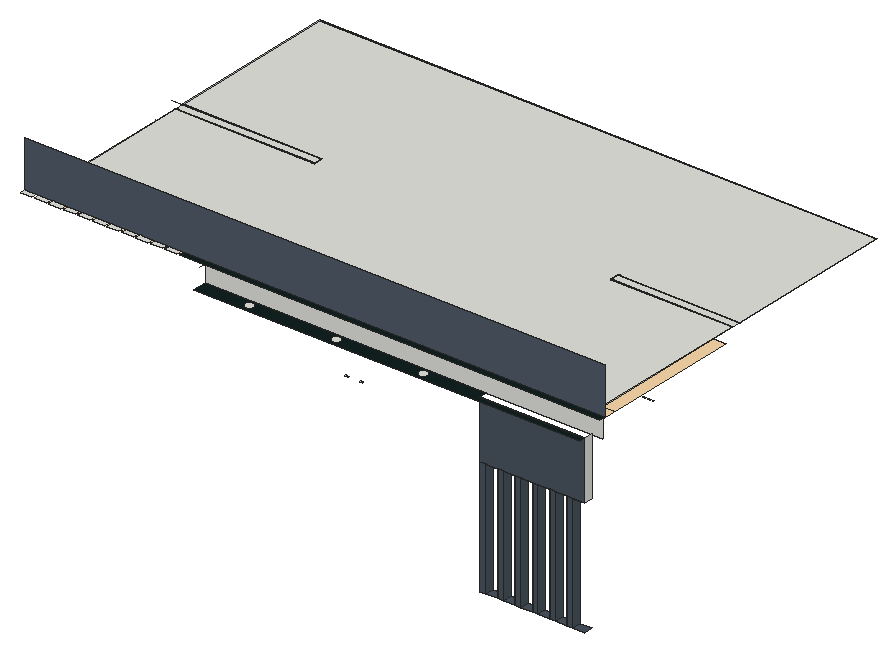
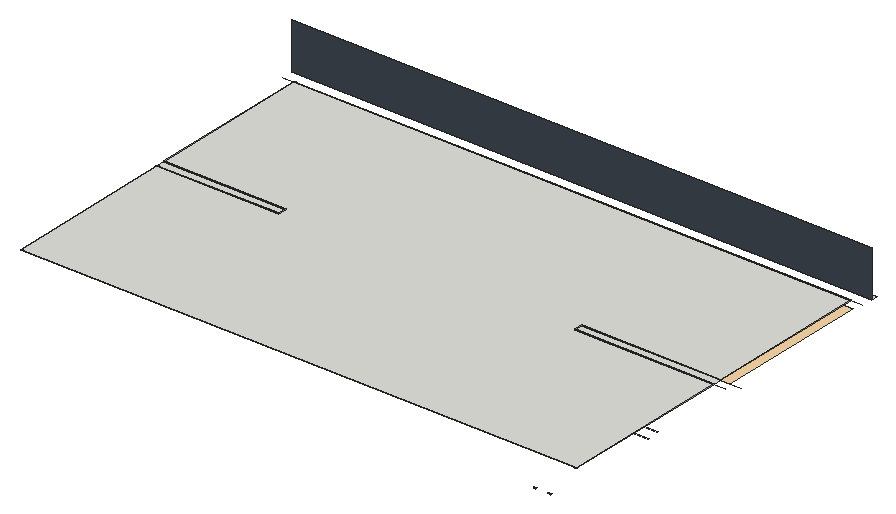
# SketchUp Ruby script. Lengths in millimetres.
U = 1.mm
M = Sketchup.active_model
def pt(a) = Geom::Point3d.new(a.map { |v| v * U })
def face(e, loops, mat)
  f = e.add_face(loops[0].map { |a| pt(a) })
  loops[1..].each { |l| e.add_face(l.map { |a| pt(a) }).erase! }
  f.material = f.back_material = mat if mat
  f
end
# faces: each face lists its corners as indices into pts; further lists are holes
def faces(e, pts, list, mat = nil) = list.each { |f| face(e, (f[0].is_a?(Array) ? f : [f]).map { |l| l.map { |i| pts[i] } }, mat) }
# xy, xz, yz: faces in a plane at the given z, y or x. An outline is a flat list of corners, or four numbers for a rectangle; further outlines are holes
def ring(l) = l.size == 4 ? [[l[0], l[1]], [l[2], l[1]], [l[2], l[3]], [l[0], l[3]]] : l.each_slice(2).to_a
def flat(e, list, mat, &to3) = list.each { |f| face(e, (f[0].is_a?(Array) ? f : [f]).map { |l| ring(l).map { |u, v| to3.(u, v) } }, mat) }
def xy(e, z, list, mat = nil) = flat(e, list, mat) { |x, y| [x, y, z] }
def xz(e, y, list, mat = nil) = flat(e, list, mat) { |x, z| [x, y, z] }
def yz(e, x, list, mat = nil) = flat(e, list, mat) { |y, z| [x, y, z] }
def lines(e, pts, list) = list.each { |a, b| e.add_line(pt(pts[a]), pt(pts[b])) }
# prism: a flat outline (further loops are holes) pulled along v
def prism(e, loops, v, mat = nil)
  f = face(e, loops, mat); d = Geom::Vector3d.new(v.map { |x| x * U })
  f.pushpull(f.normal.samedirection?(d) ? d.length : -d.length)
end
def box(e, o, s, mat = nil) = prism(e, [[o, [o[0] + s[0], o[1], o[2]], [o[0] + s[0], o[1] + s[1], o[2]], [o[0], o[1] + s[1], o[2]]]], [0, 0, s[2]], mat)
def at(x, y, z, deg = 0) = Geom::Transformation.translation(pt([x, y, z])) * Geom::Transformation.rotation(ORIGIN, Z_AXIS, deg.degrees)
def axes(o, x, y, z) = Geom::Transformation.new([*x, 0, *y, 0, *z, 0, *pt(o).to_a, 1])
def part(name) = M.definitions.add(name)
# library, detail: a bought-in or finely detailed component or shape, given as its bounding box
def library(name, o, s) = part(name).tap { |d| box(d.entities, o, s) }
def detail(e, o, s) = box(e.add_group.entities, o, s)
def put(e, d, t, mat = nil) = e.add_instance(d, t).tap { |i| i.material = mat if mat }
def group(e, t, mat = nil) = e.add_group.tap { |g| g.transformation = t; g.material = mat if mat }.entities
root = M.entities
M.materials.add("[0033_NavajoWhite]").color = [249, 217, 169]
M.materials.add("[0078_DarkSlateGray]").color = [19, 33, 33]
M.materials.add("[0110_LightSlateGray]").color = [73, 83, 94]
M.materials.add("[0111_SlateGray]").color = [81, 92, 104]
xy(root,54270.3,[[31307.7,14109.7,31917.3,14566.9],[32222.1,14109.7,32831.7,14566.9],[33136.5,14109.7,33746.1,14566.9],[34050.9,14109.7,34660.5,14566.9],[34965.3,14109.7,35574.9,14566.9],
  [35879.7,14109.7,36489.3,14566.9]],"[0110_LightSlateGray]")
xy(root,55822.5,[[17116.4,22593.3,17268.8,22644.1],[17878.4,22593.3,18030.8,22644.1]])
xy(root,60267.5,[[11965.2,22644.1,17573.6,22694.9],[17573.6,22644.1,23181.9,22694.9],[26997.1,22644.1,33251.2,22694.9]])
xy(root,60366.3,[[31307.7,14109.7,31917.3,14566.9],[32222.1,14109.7,32831.7,14566.9],[33136.5,14109.7,33746.1,14566.9],[34050.9,14109.7,34660.5,14566.9],[34965.3,14109.7,35574.9,14566.9],
  [35879.7,14109.7,36489.3,14566.9]],"[0110_LightSlateGray]")
xy(root,60755.2,[[11477.6,22644.1,23669.6,22694.9]])
xy(root,63414.3,[[18789.3,14004,18768.1,14005.1,18747.1,14008.4,18726.5,14014,18706.7,14021.6,18687.7,14031.2,18669.9,14042.8,18653.3,14056.2,18638.3,14071.2,18624.9,14087.8,18613.3,14105.6,18603.7,14124.6,18596.1,14144.4,18590.5,14165,18587.2,14186,18586.1,14207.2,18587.2,14228.4,18590.5,14249.5,18596.1,14270,18603.7,14289.9,18613.3,14308.8,18624.9,14326.6,18638.3,14343.2,18653.3,14358.2,18669.9,14371.6,18687.7,14383.2,18706.7,14392.8,18726.5,14400.5,18747.1,14406,18768.1,14409.3,18789.3,14410.4,18810.5,14409.3,18831.6,14406,18852.1,14400.5,18872,14392.8,18890.9,14383.2,18908.7,14371.6,18925.3,14358.2,18940.3,14343.2,18953.7,14326.6,18965.3,14308.8,18974.9,14289.9,18982.6,14270,18988.1,14249.5,18991.4,14228.4,18992.5,14207.2,18991.4,14186,18988.1,14165,18982.6,14144.4,18974.9,14124.6,18965.3,14105.6,18953.7,14087.8,18940.3,14071.2,18925.3,14056.2,18908.7,14042.8,18890.9,14031.2,18872,14021.6,18852.1,14014,18831.6,14008.4,18810.5,14005.1],[23361.3,14004,23340.1,14005.1,23319.1,14008.4,23298.5,14014,23278.7,14021.6,23259.7,14031.2,23241.9,14042.8,23225.3,14056.2,23210.3,14071.2,23196.9,14087.8,23185.3,14105.6,23175.7,14124.6,23168.1,14144.4,23162.5,14165,23159.2,14186,23158.1,14207.2,23159.2,14228.4,23162.5,14249.5,23168.1,14270,23175.7,14289.9,23185.3,14308.8,23196.9,14326.6,23210.3,14343.2,23225.3,14358.2,23241.9,14371.6,23259.7,14383.2,23278.7,14392.8,23298.5,14400.5,23319.1,14406,23340.1,14409.3,23361.3,14410.4,23382.5,14409.3,23403.6,14406,23424.1,14400.5,23444,14392.8,23462.9,14383.2,23480.7,14371.6,23497.3,14358.2,23512.3,14343.2,23525.7,14326.6,23537.3,14308.8,23546.9,14289.9,23554.6,14270,23560.1,14249.5,23563.4,14228.4,23564.5,14207.2,23563.4,14186,23560.1,14165,23554.6,14144.4,23546.9,14124.6,23537.3,14105.6,23525.7,14087.8,23512.3,14071.2,23497.3,14056.2,23480.7,14042.8,23462.9,14031.2,23444,14021.6,23424.1,14014,23403.6,14008.4,23382.5,14005.1],[27933.3,14004,27912.1,14005.1,27891.1,14008.4,27870.5,14014,27850.7,14021.6,27831.7,14031.2,27813.9,14042.8,27797.3,14056.2,27782.3,14071.2,27768.9,14087.8,27757.3,14105.6,27747.7,14124.6,27740.1,14144.4,27734.5,14165,27731.2,14186,27730.1,14207.2,27731.2,14228.4,27734.5,14249.5,27740.1,14270,27747.7,14289.9,27757.3,14308.8,27768.9,14326.6,27782.3,14343.2,27797.3,14358.2,27813.9,14371.6,27831.7,14383.2,27850.7,14392.8,27870.5,14400.5,27891.1,14406,27912.1,14409.3,27933.3,14410.4,27954.5,14409.3,27975.6,14406,27996.1,14400.5,28016,14392.8,28034.9,14383.2,28052.7,14371.6,28069.3,14358.2,28084.3,14343.2,28097.7,14326.6,28109.3,14308.8,28118.9,14289.9,28126.6,14270,28132.1,14249.5,28135.4,14228.4,28136.5,14207.2,28135.4,14186,28132.1,14165,28126.6,14144.4,28118.9,14124.6,28109.3,14105.6,28097.7,14087.8,28084.3,14071.2,28069.3,14056.2,28052.7,14042.8,28034.9,14031.2,28016,14021.6,27996.1,14014,27975.6,14008.4,27954.5,14005.1]])
xy(root,63414.3,[[[16220.1,13804.9,16220.1,14566.9,31002.9,14566.9,31002.9,14109.7,36489.3,14109.7,36489.3,13804.9],[23361.3,14004,23382.5,14005.1,23403.6,14008.4,23424.1,14014,23444,14021.6,23462.9,14031.2,23480.7,14042.8,23497.3,14056.2,23512.3,14071.2,23525.7,14087.8,23537.3,14105.6,23546.9,14124.6,23554.6,14144.4,23560.1,14165,23563.4,14186,23564.5,14207.2,23563.4,14228.4,23560.1,14249.5,23554.6,14270,23546.9,14289.9,23537.3,14308.8,23525.7,14326.6,23512.3,14343.2,23497.3,14358.2,23480.7,14371.6,23462.9,14383.2,23444,14392.8,23424.1,14400.5,23403.6,14406,23382.5,14409.3,23361.3,14410.4,23340.1,14409.3,23319.1,14406,23298.5,14400.5,23278.7,14392.8,23259.7,14383.2,23241.9,14371.6,23225.3,14358.2,23210.3,14343.2,23196.9,14326.6,23185.3,14308.8,23175.7,14289.9,23168.1,14270,23162.5,14249.5,23159.2,14228.4,23158.1,14207.2,23159.2,14186,23162.5,14165,23168.1,14144.4,23175.7,14124.6,23185.3,14105.6,23196.9,14087.8,23210.3,14071.2,23225.3,14056.2,23241.9,14042.8,23259.7,14031.2,23278.7,14021.6,23298.5,14014,23319.1,14008.4,23340.1,14005.1],[27933.3,14004,27954.5,14005.1,27975.6,14008.4,27996.1,14014,28016,14021.6,28034.9,14031.2,28052.7,14042.8,28069.3,14056.2,28084.3,14071.2,28097.7,14087.8,28109.3,14105.6,28118.9,14124.6,28126.6,14144.4,28132.1,14165,28135.4,14186,28136.5,14207.2,28135.4,14228.4,28132.1,14249.5,28126.6,14270,28118.9,14289.9,28109.3,14308.8,28097.7,14326.6,28084.3,14343.2,28069.3,14358.2,28052.7,14371.6,28034.9,14383.2,28016,14392.8,27996.1,14400.5,27975.6,14406,27954.5,14409.3,27933.3,14410.4,27912.1,14409.3,27891.1,14406,27870.5,14400.5,27850.7,14392.8,27831.7,14383.2,27813.9,14371.6,27797.3,14358.2,27782.3,14343.2,27768.9,14326.6,27757.3,14308.8,27747.7,14289.9,27740.1,14270,27734.5,14249.5,27731.2,14228.4,27730.1,14207.2,27731.2,14186,27734.5,14165,27740.1,14144.4,27747.7,14124.6,27757.3,14105.6,27768.9,14087.8,27782.3,14071.2,27797.3,14056.2,27813.9,14042.8,27831.7,14031.2,27850.7,14021.6,27870.5,14014,27891.1,14008.4,27912.1,14005.1],[18789.3,14004,18810.5,14005.1,18831.6,14008.4,18852.1,14014,18872,14021.6,18890.9,14031.2,18908.7,14042.8,18925.3,14056.2,18940.3,14071.2,18953.7,14087.8,18965.3,14105.6,18974.9,14124.6,18982.6,14144.4,18988.1,14165,18991.4,14186,18992.5,14207.2,18991.4,14228.4,18988.1,14249.5,18982.6,14270,18974.9,14289.9,18965.3,14308.8,18953.7,14326.6,18940.3,14343.2,18925.3,14358.2,18908.7,14371.6,18890.9,14383.2,18872,14392.8,18852.1,14400.5,18831.6,14406,18810.5,14409.3,18789.3,14410.4,18768.1,14409.3,18747.1,14406,18726.5,14400.5,18706.7,14392.8,18687.7,14383.2,18669.9,14371.6,18653.3,14358.2,18638.3,14343.2,18624.9,14326.6,18613.3,14308.8,18603.7,14289.9,18596.1,14270,18590.5,14249.5,18587.2,14228.4,18586.1,14207.2,18587.2,14186,18590.5,14165,18596.1,14144.4,18603.7,14124.6,18613.3,14105.6,18624.9,14087.8,18638.3,14071.2,18653.3,14056.2,18669.9,14042.8,18687.7,14031.2,18706.7,14021.6,18726.5,14014,18747.1,14008.4,18768.1,14005.1]]],"[0078_DarkSlateGray]")
xy(root,64328.7,[[7685.7,14566.9,37098.9,22644.1]],"[0033_NavajoWhite]")
xy(root,64785.9,[[7076.1,13804.9,7685.7,14109.7],[7838.1,13804.9,8447.7,14109.7],[8600.1,13804.9,9209.7,14109.7],[9362.1,13804.9,9971.7,14109.7],[10124.1,13804.9,10733.7,14109.7],
  [10886.1,13804.9,11495.7,14109.7],[11648.1,13804.9,12257.7,14109.7],[12410.1,13804.9,13019.7,14109.7],[13172.1,13804.9,13781.7,14109.7],[13934.1,13804.9,14543.7,14109.7],
  [14696.1,13804.9,15305.7,14109.7],[7685.7,14719.3,7685.7,23253.7,15000.9,23253.7,15000.9,23710.9,7685.7,23710.9,7685.7,32702.5,36946.5,32702.5,36946.5,23710.9,30545.7,23710.9,30545.7,23253.7,36946.5,23253.7,36946.5,14719.3],[7685.7,23253.7,15000.9,23710.9],[30545.7,23253.7,36946.5,23710.9]])
xy(root,64785.9,[[15458.1,13804.9,37556.1,14109.7]],"[0078_DarkSlateGray]")
xz(root,14109.7,[[31002.9,54270.3,31307.7,60366.3],[31917.3,54270.3,32222.1,60366.3],[32831.7,54270.3,33136.5,60366.3],[33746.1,54270.3,34050.9,60366.3],[34660.5,54270.3,34965.3,60366.3],
  [35574.9,54270.3,35879.7,60366.3],[31002.9,60366.3,36489.3,63414.3]],"[0110_LightSlateGray]")
xz(root,14109.7,[[7076.1,64785.9,37556.1,67224.3]],"[0111_SlateGray]")
xz(root,14566.9,[[16220.1,63414.3,37098.9,64328.7]])
xz(root,14719.3,[[7685.7,64785.9,36946.5,64811.3]])
xz(root,23253.7,[[7685.7,64785.9,15000.9,64811.3],[30545.7,64785.9,36946.5,64811.3]])
xz(root,23710.9,[[7685.7,64785.9,15000.9,64811.3],[30545.7,64785.9,36946.5,64811.3]])
xz(root,32702.5,[[7685.7,64785.9,36946.5,64811.3]])
yz(root,7685.7,[[14719.3,64785.9,23253.7,64811.3],[23710.9,64785.9,32702.5,64811.3]])
yz(root,15000.9,[[23253.7,64785.9,23710.9,64811.3]])
yz(root,30545.7,[[23253.7,64785.9,23710.9,64811.3]])
yz(root,31307.7,[[14109.7,54270.3,14566.9,60366.3]],"[0110_LightSlateGray]")
yz(root,31917.3,[[14109.7,54270.3,14566.9,60366.3]],"[0110_LightSlateGray]")
yz(root,32222.1,[[14109.7,54270.3,14566.9,60366.3]],"[0110_LightSlateGray]")
yz(root,32831.7,[[14109.7,54270.3,14566.9,60366.3]],"[0110_LightSlateGray]")
yz(root,33136.5,[[14109.7,54270.3,14566.9,60366.3]],"[0110_LightSlateGray]")
yz(root,33746.1,[[14109.7,54270.3,14566.9,60366.3]],"[0110_LightSlateGray]")
yz(root,34050.9,[[14109.7,54270.3,14566.9,60366.3]],"[0110_LightSlateGray]")
yz(root,34660.5,[[14109.7,54270.3,14566.9,60366.3]],"[0110_LightSlateGray]")
yz(root,34965.3,[[14109.7,54270.3,14566.9,60366.3]],"[0110_LightSlateGray]")
yz(root,35574.9,[[14109.7,54270.3,14566.9,60366.3]],"[0110_LightSlateGray]")
yz(root,35879.7,[[14109.7,54270.3,14566.9,60366.3]],"[0110_LightSlateGray]")
yz(root,36489.3,[[14109.7,60366.3,14566.9,63414.3]])
yz(root,36946.5,[[14719.3,64785.9,23253.7,64811.3],[23710.9,64785.9,32702.5,64811.3]])
p = [[7685.7,22644.1,64328.7],[7076.1,22644.1,64328.7],[16220.1,14566.9,64328.7],[16220.1,14109.7,64328.7],[7685.7,23710.9,64785.9],[7076.1,23710.9,64785.9],
  [7685.7,14719.3,64785.9],[7076.1,14719.3,64785.9],[36946.5,14719.3,64785.9],[37556.1,14719.3,64785.9]]
lines(root,p,[[0,1],[2,3],[4,5],[6,7],[8,9]])
